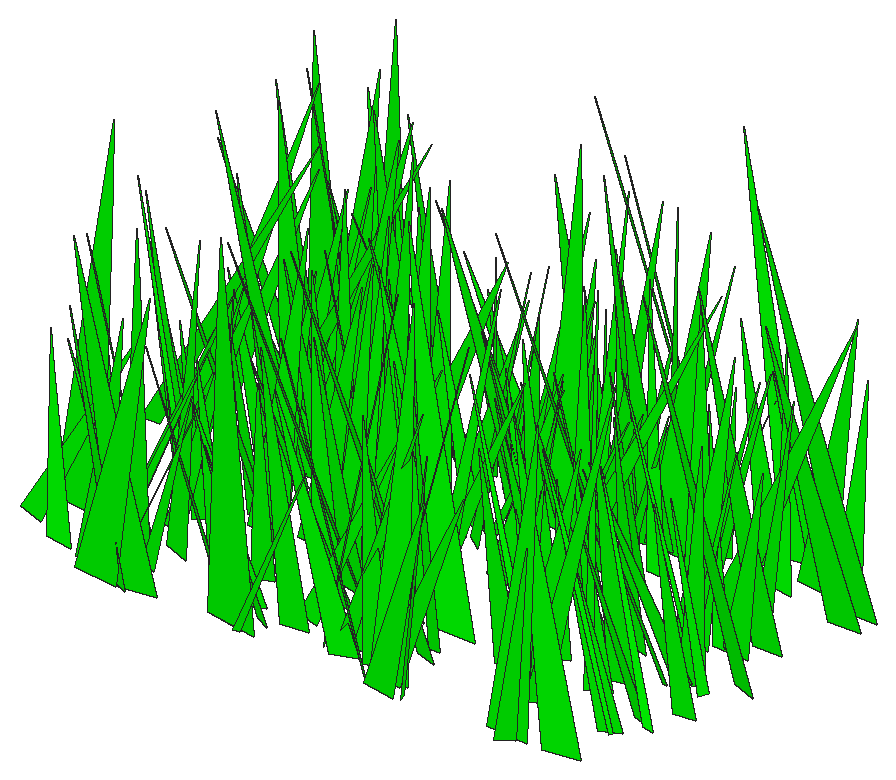
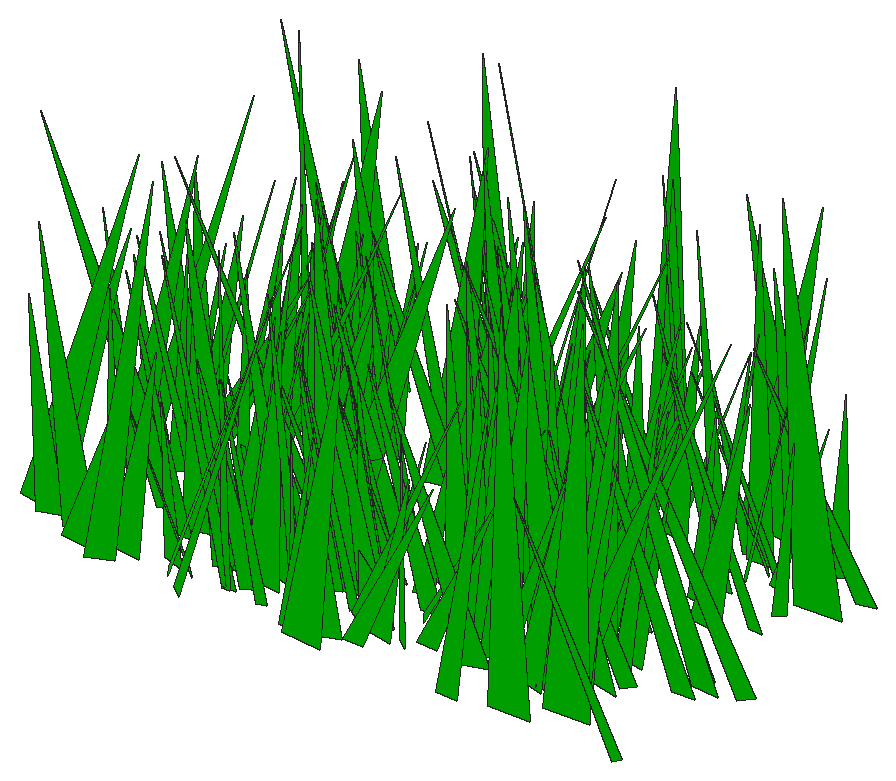
# SketchUp Ruby script. Lengths in inches.
U = 1.inch
M = Sketchup.active_model
def pt(a) = Geom::Point3d.new(a.map { |v| v * U })
def face(e, loops, mat)
  f = e.add_face(loops[0].map { |a| pt(a) })
  loops[1..].each { |l| e.add_face(l.map { |a| pt(a) }).erase! }
  f.material = f.back_material = mat if mat
  f
end
# faces: each face lists its corners as indices into pts; further lists are holes
def faces(e, pts, list, mat = nil) = list.each { |f| face(e, (f[0].is_a?(Array) ? f : [f]).map { |l| l.map { |i| pts[i] } }, mat) }
# xy, xz, yz: faces in a plane at the given z, y or x. An outline is a flat list of corners, or four numbers for a rectangle; further outlines are holes
def ring(l) = l.size == 4 ? [[l[0], l[1]], [l[2], l[1]], [l[2], l[3]], [l[0], l[3]]] : l.each_slice(2).to_a
def flat(e, list, mat, &to3) = list.each { |f| face(e, (f[0].is_a?(Array) ? f : [f]).map { |l| ring(l).map { |u, v| to3.(u, v) } }, mat) }
def xy(e, z, list, mat = nil) = flat(e, list, mat) { |x, y| [x, y, z] }
def xz(e, y, list, mat = nil) = flat(e, list, mat) { |x, z| [x, y, z] }
def yz(e, x, list, mat = nil) = flat(e, list, mat) { |y, z| [x, y, z] }
def lines(e, pts, list) = list.each { |a, b| e.add_line(pt(pts[a]), pt(pts[b])) }
# prism: a flat outline (further loops are holes) pulled along v
def prism(e, loops, v, mat = nil)
  f = face(e, loops, mat); d = Geom::Vector3d.new(v.map { |x| x * U })
  f.pushpull(f.normal.samedirection?(d) ? d.length : -d.length)
end
def box(e, o, s, mat = nil) = prism(e, [[o, [o[0] + s[0], o[1], o[2]], [o[0] + s[0], o[1] + s[1], o[2]], [o[0], o[1] + s[1], o[2]]]], [0, 0, s[2]], mat)
def at(x, y, z, deg = 0) = Geom::Transformation.translation(pt([x, y, z])) * Geom::Transformation.rotation(ORIGIN, Z_AXIS, deg.degrees)
def axes(o, x, y, z) = Geom::Transformation.new([*x, 0, *y, 0, *z, 0, *pt(o).to_a, 1])
def part(name) = M.definitions.add(name)
# library, detail: a bought-in or finely detailed component or shape, given as its bounding box
def library(name, o, s) = part(name).tap { |d| box(d.entities, o, s) }
def detail(e, o, s) = box(e.add_group.entities, o, s)
def put(e, d, t, mat = nil) = e.add_instance(d, t).tap { |i| i.material = mat if mat }
def group(e, t, mat = nil) = e.add_group.tap { |g| g.transformation = t; g.material = mat if mat }.entities
root = M.entities
M.materials.add("[0065_Lime]").color = [0, 255, 0]
c1 = part("fur_instance\#9")
p = [[0.8125,0,1.79],[0.67,-0.02,1.48],[0,-0.11,0],[0,0.11,0]]
faces(c1.entities,p,[[0,1,2,3]])
put(root,c1,axes([28.72,22.77,1.48],[-3.5361,0.35357,0.62096],[-2.38381,-0.50693,0.69047],[1.10969,0.03769,3.46199]),"[0065_Lime]")
put(root,c1,axes([28.78,19.72,1.48],[-2.9775,0.57338,0.01359],[-3.98278,-0.409,0.88436],[0.88789,0.0882,4.01253]),"[0065_Lime]")
put(root,c1,axes([27.87,21.88,1.48],[1.59134,1.15221,2.92207],[-8.95191,0.2009,0.57103],[0.06821,-0.51425,6.7702]),"[0065_Lime]")
put(root,c1,axes([29.9,21.47,1.48],[-3.74921,0.205,0.84488],[-1.69704,-0.51484,-0.79677],[0.572,-0.18381,3.17391]),"[0065_Lime]")
put(root,c1,axes([26.9,33.24,1.48],[5.29508,-0.1762,0.18665],[1.27098,0.7403,-0.43903],[-0.09771,0.08126,4.40438]),"[0065_Lime]")
put(root,c1,axes([26.95,20.6,1.48],[3.52402,0.60278,0.02909],[-4.2165,0.4855,0.855],[0.78993,-0.09757,4.43406]),"[0065_Lime]")
put(root,c1,axes([30.1,24.78,1.48],[-1.53905,0.72746,1.23673],[-5.38247,-0.19147,-0.65785],[-0.37698,-0.23612,4.34366]),"[0065_Lime]")
put(root,c1,axes([30.03,24.65,1.48],[-4.90512,-0.53874,1.71755],[4.17986,-0.70878,0.44836],[1.29866,0.24644,5.04419]),"[0065_Lime]")
put(root,c1,axes([30.4375,24.15,1.48],[-6.75899,0.10318,1.4523],[-0.56299,-0.97914,0.59733],[1.84661,0.07913,5.49784]),"[0065_Lime]")
put(root,c1,axes([27.95,27.57,1.48],[1.90571,-0.57874,0.3586],[4.07605,0.24988,-0.81846],[0.73696,0.11448,3.5995]),"[0065_Lime]")
put(root,c1,axes([30.14,31.13,1.48],[-4.8108,0.36742,1.63412],[-3.00649,-0.69382,-0.62879],[1.35421,-0.23512,4.40921]),"[0065_Lime]")
put(root,c1,axes([31.47,29.57,1.48],[-4.36689,-0.72132,0.39514],[5.15363,-0.60775,0.50828],[-0.16377,0.10881,5.45836]),"[0065_Lime]")
put(root,c1,axes([26.15,27.65,1.48],[8.05448,-0.36593,0.10917],[2.60265,1.12434,-0.76218],[0.16139,0.13106,6.84324]),"[0065_Lime]")
put(root,c1,axes([30.34,28.14,1.48],[-2.77665,0.35489,1.36449],[-2.98789,-0.37458,-0.75831],[0.51496,-0.25978,2.95745]),"[0065_Lime]")
put(root,c1,axes([30.97,21.69,1.48],[-6.33616,-0.14954,1.16675],[0.98148,-0.9122,-0.39106],[1.49221,-0.03497,5.21145]),"[0065_Lime]")
put(root,c1,axes([30.48,28.47,1.48],[-4.82918,-0.53417,1.11755],[3.75382,-0.70422,-0.54689],[1.4992,0.04263,4.96915]),"[0065_Lime]")
put(root,c1,axes([30.53,30.6,1.48],[-5.41771,-0.76266,1.43966],[5.44632,-0.79326,-0.52083],[1.7111,0.11017,6.21606]),"[0065_Lime]")
put(root,c1,axes([27.85,28.6875,1.48],[5.15808,0.64552,0.65599],[-4.66345,0.71658,0.63311],[-0.07723,-0.15712,5.58261]),"[0065_Lime]")
put(root,c1,axes([29.92,32,1.48],[-1.86684,-1.23711,0.9246],[8.83963,-0.27404,-0.47748],[0.81409,0.13867,7.30489]),"[0065_Lime]")
put(root,c1,axes([27.49,28.05,1.48],[7.17751,0.78944,0.96843],[-5.7172,1.00753,0.51447],[-0.54212,-0.17345,7.39622]),"[0065_Lime]")
put(root,c1,axes([28.67,24.05,1.48],[5.56756,-0.25053,0.07454],[1.75703,0.77643,0.61209],[-0.31607,-0.09682,4.7157]),"[0065_Lime]")
put(root,c1,axes([32.28,27.27,1.48],[-5.81157,-0.70001,1.7086],[5.33705,-0.81199,0.86353],[0.86294,0.30768,6.16607]),"[0065_Lime]")
put(root,c1,axes([30.13,29.91,1.48],[3.34774,0.73264,0.07321],[-5.18012,0.46896,-0.5325],[-0.59929,0.03912,5.0118]),"[0065_Lime]")
put(root,c1,axes([31.3125,23.7,1.48],[-3.40261,0.29121,1.77597],[-2.75556,-0.48772,-0.81322],[1.212,-0.2913,3.137]),"[0065_Lime]")
put(root,c1,axes([31.93,18.76,1.48],[-5.23082,-0.46131,0.97469],[3.16859,-0.75388,-0.70499],[1.47422,-0.01646,4.97365]),"[0065_Lime]")
put(root,c1,axes([32.09,31.2,1.48],[-2.31985,-0.60177,1.93],[4.89532,-0.29083,0.85459],[0.07595,0.36448,3.86846]),"[0065_Lime]")
put(root,c1,axes([30.48,19.34,1.48],[1.0224,-0.87725,0.57335],[6.26705,0.13534,-0.45547],[0.44254,0.11016,5.12558]),"[0065_Lime]")
put(root,c1,axes([32.7,30.59,1.48],[-7.74786,-0.11969,1.71735],[1.11795,-1.11673,0.72901],[1.98325,0.1619,6.29814]),"[0065_Lime]")
put(root,c1,axes([31.26,20.54,1.48],[4.80827,0.64677,3.01034],[-5.54314,0.72565,0.63379],[-2.03855,-0.44763,5.37703]),"[0065_Lime]")
put(root,c1,axes([32.66,18.77,1.48],[-1.21146,-1.0565,1.5288],[7.71905,-0.14063,0.79057],[-0.6918,0.28098,6.14398]),"[0065_Lime]")
put(root,c1,axes([32.08,27.91,1.48],[0.92743,-1.10638,2.25257],[8.30169,0.16274,0.41694],[-0.8625,0.37673,6.43525]),"[0065_Lime]")
put(root,c1,axes([33.12,31.41,1.48],[-4.13307,-0.46976,1.03758],[3.56684,-0.56267,0.86424],[0.2846,0.22982,4.23675]),"[0065_Lime]")
put(root,c1,axes([31.43,33.01,1.48],[-3.49602,-1.09361,2.3833],[8.09772,-0.54934,-0.58752],[1.89292,0.33024,6.91506]),"[0065_Lime]")
put(root,c1,axes([30.59,30.26,1.48],[5.59751,-0.2494,1.37056],[2.08303,0.79577,-0.77659],[-1.28457,0.20365,4.71293]),"[0065_Lime]")
put(root,c1,axes([33.59,27.43,1.48],[-2.81131,0.48483,0.02706],[-3.36983,-0.38449,-0.79968],[-0.74168,-0.0908,3.53078]),"[0065_Lime]")
put(root,c1,axes([30.1,21.04,1.48],[4.99048,0.28877,0.35872],[-2.08973,0.6988,0.3855],[-0.22515,-0.08529,4.37307]),"[0065_Lime]")
put(root,c1,axes([34.15,23.88,1.48],[-6.14823,-0.31663,0.55577],[2.32834,-0.85754,0.67122],[0.35091,0.14224,5.28389]),"[0065_Lime]")
put(root,c1,axes([30.93,31.15,1.48],[5.00355,-1.08655,0.74643],[7.72341,0.71202,0.47601],[-0.99127,0.06314,7.47653]),"[0065_Lime]")
put(root,c1,axes([30.68,20.86,1.48],[4.29098,0.08918,0.19069],[-0.58149,0.59423,-0.65508],[-0.34589,0.10737,3.46697]),"[0065_Lime]")
put(root,c1,axes([32.72,24.77,1.48],[-2.80205,-0.50191,0.49495],[3.53201,-0.40248,-0.44632],[0.80839,0.01877,3.66567]),"[0065_Lime]")
put(root,c1,axes([31.55,26.2,1.48],[0.82876,0.56028,0.01444],[-3.94864,0.11497,0.46315],[0.55391,-0.0187,3.28007]),"[0065_Lime]")
put(root,c1,axes([31.07,18.71,1.48],[1.54058,-1.05232,0.3585],[7.45525,0.20773,-0.7651],[0.83471,0.08688,6.17187]),"[0065_Lime]")
put(root,c1,axes([31.14,22.58,1.48],[4.95946,0.50295,1.09358],[-3.75844,0.6981,0.51904],[-0.70189,-0.1844,4.9478]),"[0065_Lime]")
put(root,c1,axes([32.09,21.51,1.48],[5.68742,0.51625,2.39145],[-4.26718,0.83899,0.64564],[-1.98301,-0.32476,5.46951]),"[0065_Lime]")
put(root,c1,axes([31.9375,20.31,1.48],[3.62474,0.29569,1.03947],[-2.38327,0.50159,0.71752],[-0.61742,-0.20021,3.33288]),"[0065_Lime]")
put(root,c1,axes([29.53,29.36,1.48],[8.42142,-0.30369,0.21284],[2.17439,1.18058,-0.47674],[-0.10711,0.08893,7.05599]),"[0065_Lime]")
put(root,c1,axes([33.83,30.46,1.48],[-4.81529,0.95459,0.64171],[-6.73172,-0.68549,0.74786],[1.20687,-0.01484,6.73179]),"[0065_Lime]")
put(root,c1,axes([33.67,33.36,1.48],[-5.15186,-0.62922,1.2017],[4.44942,-0.7505,-0.54693],[1.56092,0.06256,5.52527]),"[0065_Lime]")
put(root,c1,axes([34.57,20.59,1.48],[-4.89615,-0.12504,0.52726],[0.96937,-0.68647,0.50055],[0.5219,0.10196,4.01677]),"[0065_Lime]")
put(root,c1,axes([31.49,29.89,1.48],[5.60129,-0.86407,1.25797],[6.32205,0.78329,-0.59656],[-0.4859,0.23062,6.73952]),"[0065_Lime]")
put(root,c1,axes([32.66,25.73,1.48],[-1.28123,0.7327,1.5636],[-5.36847,-0.23483,0.77688],[1.43652,-0.22411,4.29789]),"[0065_Lime]")
put(root,c1,axes([33.58,28.07,1.48],[-3.70234,-0.61665,2.81856],[5.36388,-0.55661,0.58114],[1.57923,0.44487,4.63397]),"[0065_Lime]")
put(root,c1,axes([34.47,20.88,1.48],[1.58425,-0.6212,1.32415],[4.55005,0.26431,0.55305],[-1.22082,0.17896,3.7796]),"[0065_Lime]")
put(root,c1,axes([33.56,24.29,1.48],[0.88439,0.99039,1.1984],[-7.19374,0.11248,0.39757],[0.31229,-0.21366,5.76435]),"[0065_Lime]")
put(root,c1,axes([35.39,25.48,1.48],[-2.98273,-0.68462,1.34787],[5.14146,-0.40797,0.58425],[0.22049,0.25188,4.60985]),"[0065_Lime]")
put(root,c1,axes([33.07,28.9,1.48],[5.33723,-0.97526,0.63904],[6.9226,0.75708,0.46229],[-0.93024,0.03845,7.10671]),"[0065_Lime]")
put(root,c1,axes([34.9375,29.76,1.48],[-4.28948,0.66055,0.95634],[-4.63171,-0.62376,0.69147],[1.42395,-0.03907,5.12999]),"[0065_Lime]")
put(root,c1,axes([36.16,31.25,1.48],[-2.88799,0.47312,0.00249],[-3.34241,-0.40279,-0.4371],[-0.4059,-0.04948,3.58162]),"[0065_Lime]")
put(root,c1,axes([37.38,29.875,1.48],[-5.94972,-0.10522,0.01679],[0.74009,-0.82214,0.88385],[-0.11554,0.15185,4.79701]),"[0065_Lime]")
put(root,c1,axes([36.27,20.35,1.48],[-2.32592,0.50491,0.2701],[-3.57596,-0.31507,-0.6386],[-0.48366,-0.09863,3.42259]),"[0065_Lime]")
put(root,c1,axes([36.1,26.7,1.48],[-5.8963,-0.11837,1.20908],[0.5988,-0.84605,-0.84341],[1.60016,-0.11957,4.77085]),"[0065_Lime]")
put(root,c1,axes([35.86,28.8125,1.48],[0.5666,-1.20776,1.69318],[8.79229,0.10843,0.6451],[-0.95048,0.28308,6.97674]),"[0065_Lime]")
put(root,c1,axes([35.75,29.3,1.48],[1.10258,0.92393,0.21284],[-6.52192,0.15839,-0.68613],[-0.87547,-0.01635,5.37946]),"[0065_Lime]")
put(root,c1,axes([35.31,21.86,1.48],[2.47408,-0.61407,0.28859],[4.26838,0.35042,0.77422],[-1.00197,-0.02346,4.01073]),"[0065_Lime]")
put(root,c1,axes([35.86,28.45,1.48],[-4.21318,0.26406,1.69127],[-2.32385,-0.62403,-0.56551],[1.56659,-0.21552,3.70963]),"[0065_Lime]")
put(root,c1,axes([35.46,19.21,1.48],[6.90338,0.01171,2.27071],[0.22301,1.04031,-0.62834],[-2.78391,0.11237,5.58045]),"[0065_Lime]")
put(root,c1,axes([38.28,23.01,1.48],[-7.29496,-0.31664,0.22657],[2.2031,-1.01897,-0.78601],[0.54938,-0.11836,6.16053]),"[0065_Lime]")
put(root,c1,axes([34.12,31.34,1.48],[3.2239,-0.67529,0.07675],[4.76102,0.44643,-0.69802],[0.66075,0.07807,4.65512]),"[0065_Lime]")
put(root,c1,axes([37.03,19.67,1.48],[-3.52449,-0.30166,0.04655],[2.08957,-0.48527,-0.70038],[0.49576,-0.09925,3.28295]),"[0065_Lime]")
put(root,c1,axes([36.37,23.83,1.48],[-3.33471,0.69059,2.37133],[-5.58773,-0.49334,-0.38478],[1.19562,-0.37948,4.81564]),"[0065_Lime]")
put(root,c1,axes([36.03,19.03,1.48],[-2.69771,-0.90102,1.5194],[6.53677,-0.41426,-0.55272],[1.36942,0.20244,5.63147]),"[0065_Lime]")
put(root,c1,axes([35.21,24.59,1.48],[0.24312,-0.82666,1.95285],[6.27852,-0.02063,-0.80985],[0.97658,0.33845,4.72042]),"[0065_Lime]")
put(root,c1,axes([38.11,32.52,1.48],[-3.39189,0.46363,0.00651],[-3.27769,-0.47329,-0.44778],[-0.37814,-0.05623,3.82288]),"[0065_Lime]")
put(root,c1,axes([36.3,18.99,1.48],[-3.07127,-1.23304,1.14461],[8.75798,-0.45547,-0.89295],[1.50956,0.13379,7.50937]),"[0065_Lime]")
put(root,c1,axes([36.33,29.25,1.48],[-4.4804,0.75461,1.72832],[-5.34027,-0.6852,0.86516],[2.19892,-0.12652,5.62266]),"[0065_Lime]")
put(root,c1,axes([38.12,27.9,1.48],[-3.33452,-0.74369,0.8425],[5.38721,-0.45149,0.75292],[-0.24776,0.19206,5.03218]),"[0065_Lime]")
put(root,c1,axes([36.35,28,1.48],[5.99666,0.08389,1.90852],[-0.21962,0.89588,-0.86292],[-2.41108,0.12703,4.82532]),"[0065_Lime]")
put(root,c1,axes([38.42,22.09,1.48],[-3.87251,-0.50419,0.22774],[3.5912,-0.53754,0.52601],[-0.2363,0.09329,4.26187]),"[0065_Lime]")
put(root,c1,axes([36.45,27.32,1.48],[4.57674,0.51359,2.35356],[-4.2925,0.68652,0.50284],[-1.81804,-0.32801,4.73762]),"[0065_Lime]")
put(root,c1,axes([36.83,31.64,1.48],[4.25887,0.2267,1.4966],[-1.40147,0.65138,-0.66749],[-2.00595,0.02621,3.64381]),"[0065_Lime]")
put(root,c1,axes([36.5,27.79,1.48],[-3.589,0.86041,2.2665],[-6.42175,-0.5704,0.52778],[2.00448,-0.28685,5.74898]),"[0065_Lime]")
put(root,c1,axes([39.02,31.23,1.48],[-5.80078,-0.31348,0.56422],[2.32259,-0.80199,0.86783],[0.25245,0.17526,4.9803]),"[0065_Lime]")
put(root,c1,axes([37.71,31.74,1.48],[0.30036,0.57934,0.57781],[-4.07128,0.06351,-0.73363],[-0.96309,-0.08781,3.2815]),"[0065_Lime]")
put(root,c1,axes([38.02,20.04,1.48],[1.81678,0.74005,1.96243],[-5.56498,0.32164,-0.65572],[-1.60892,-0.27685,4.48395]),"[0065_Lime]")
put(root,c1,axes([38.35,28.68,1.48],[-3.14554,0.50459,0.05274],[-3.56846,-0.44046,0.39336],[0.4063,0.03796,3.8631]),"[0065_Lime]")
put(root,c1,axes([36.89,24.62,1.48],[-6.25067,0.53072,2.74807],[-3.7036,-0.99297,0.85218],[3.45864,-0.10414,5.87903]),"[0065_Lime]")
put(root,c1,axes([38.07,23.05,1.48],[-3.58353,-0.68054,0.41693],[4.77266,-0.50853,-0.67321],[0.9697,-0.01207,4.85414]),"[0065_Lime]")
put(root,c1,axes([36.9,23.99,1.48],[5.49947,-0.68316,1.31727],[4.8466,0.80183,0.54675],[-1.66411,0.07762,5.94563]),"[0065_Lime]")
put(root,c1,axes([37.44,25.22,1.48],[5.56364,1.01805,1.63954],[-7.2201,0.82166,-0.88547],[-2.10305,-0.12763,7.37739]),"[0065_Lime]")
put(root,c1,axes([38.96,29.94,1.48],[-3.5513,-0.26544,0.96159],[2.14498,-0.49191,0.69119],[0.60421,0.18613,3.19809]),"[0065_Lime]")
put(root,c1,axes([36.7,18.79,1.48],[4.27715,-0.09296,0.41345],[0.72331,0.59911,-0.43702],[-0.41574,0.08595,3.49323]),"[0065_Lime]")
put(root,c1,axes([40.58,23.0625,1.48],[-7.29683,-0.44608,0.32237],[3.12189,-1.02315,-0.6878],[0.6991,-0.087,6.43607]),"[0065_Lime]")
put(root,c1,axes([37.37,29.47,1.48],[2.83428,0.62215,0.79426],[-4.5335,0.38652,0.55846],[0.0662,-0.16747,4.23954]),"[0065_Lime]")
put(root,c1,axes([37.67,31.07,1.48],[5.36353,0.10664,1.19403],[-0.93308,0.77362,0.45793],[-1.36386,-0.1099,4.38236]),"[0065_Lime]")
put(root,c1,axes([36.97,24.11,1.48],[1.97069,0.7444,0.07462],[-5.20422,0.26938,0.89002],[0.99427,-0.06547,4.51063]),"[0065_Lime]")
put(root,c1,axes([40.37,19.63,1.48],[-1.89031,0.76108,0.06694],[-5.33542,-0.25948,-0.82906],[-0.93573,-0.05794,4.592]),"[0065_Lime]")
put(root,c1,axes([39.49,33.44,1.48],[0.22938,-0.98535,0.85706],[7.04804,0.04796,0.59973],[-0.77943,0.14373,5.67534]),"[0065_Lime]")
put(root,c1,axes([40.875,23.74,1.48],[-2.69535,0.98539,0.29612],[-7.01004,-0.37438,-0.47069],[-0.41055,-0.07681,6.09282]),"[0065_Lime]")
put(root,c1,axes([38.91,32.72,1.48],[-2.82008,0.53735,1.9113],[-4.06504,-0.4711,0.46973],[1.90276,-0.21004,3.83627]),"[0065_Lime]")
put(root,c1,axes([39.22,30.2,1.48],[-0.60579,-0.66776,0.84299],[4.80927,-0.10416,-0.47813],[0.72663,0.13268,3.86731]),"[0065_Lime]")
put(root,c1,axes([37.99,20.77,1.48],[3.76153,0.52015,0.16729],[-3.69528,0.52271,0.51501],[0.2989,-0.08358,4.26172]),"[0065_Lime]")
put(root,c1,axes([40.68,23.66,1.48],[-2.04476,0.66088,1.10482],[-4.89536,-0.27592,-0.46396],[-0.00293,-0.207,4.14565]),"[0065_Lime]")
put(root,c1,axes([41.6875,19.02,1.48],[-6.95907,-0.05614,1.00741],[0.56116,-0.98368,0.72806],[1.17412,0.13742,5.62298]),"[0065_Lime]")
put(root,c1,axes([40.47,33.04,1.48],[-4.02546,0.1987,1.20461],[-1.64443,-0.5872,-0.39031],[1.22004,-0.13587,3.44848]),"[0065_Lime]")
put(root,c1,axes([39.01,27.89,1.48],[6.34506,0.23684,1.53199],[-2.01871,0.90522,0.84266],[-1.52079,-0.21346,5.27324]),"[0065_Lime]")
put(root,c1,axes([40.08,33.06,1.48],[-3.58682,-0.28311,1.22965],[1.72526,-0.54544,-0.87832],[1.8352,-0.04055,3.229]),"[0065_Lime]")
put(root,c1,axes([39.38,30.05,1.48],[4.93183,0.80591,0.77487],[-5.71705,0.70416,-0.46525],[-1.05643,-0.04839,6.13515]),"[0065_Lime]")
put(root,c1,axes([39.42,30.84,1.48],[5.01325,-0.13726,1.02114],[1.1167,0.71909,-0.38842],[-1.13276,0.10141,4.13633]),"[0065_Lime]")
put(root,c1,axes([39.22,28.55,1.48],[3.98991,0.17878,0.30958],[-1.31259,0.55662,0.42183],[-0.20162,-0.08584,3.38023]),"[0065_Lime]")
put(root,c1,axes([42.14,22.83,1.48],[-4.68194,1.13728,0.03042],[-8.06271,-0.65591,0.64589],[0.706,0.05134,7.57804]),"[0065_Lime]")
put(root,c1,axes([40.32,32.46,1.48],[6.59305,-0.1941,2.1072],[1.75501,0.97795,-0.61461],[-2.35351,0.18551,5.44473]),"[0065_Lime]")
put(root,c1,axes([39.32,19.96,1.48],[8.53091,0.06369,1.77067],[-0.7424,1.22477,0.89031],[-2.09593,-0.17459,6.89167]),"[0065_Lime]")
put(root,c1,axes([40.68,30.18,1.48],[-3.98422,1.03163,2.37649],[-7.61061,-0.62465,0.64425],[2.12476,-0.30297,6.7639]),"[0065_Lime]")
put(root,c1,axes([43.13,26.73,1.48],[-4.6572,-0.95591,0.9855],[6.90582,-0.63696,0.88985],[-0.23403,0.22701,6.64664]),"[0065_Lime]")
put(root,c1,axes([40.21,28.1875,1.48],[-0.11964,-0.56067,1.10236],[4.09221,-0.06092,-0.74433],[1.00548,0.18121,3.16056]),"[0065_Lime]")
put(root,c1,axes([40.83,20.19,1.48],[-1.21884,0.633,0.29729],[-4.41637,-0.17811,0.72802],[0.96029,-0.01571,3.72552]),"[0065_Lime]")
put(root,c1,axes([40.71,30.3,1.48],[-3.04412,0.45262,1.80916],[-3.29809,-0.50982,0.60221],[2.10826,-0.144,3.55433]),"[0065_Lime]")
put(root,c1,axes([41.61,19.77,1.48],[2.65298,-0.698,1.21069],[4.99553,0.40703,0.62062],[-1.39085,0.13054,4.53842]),"[0065_Lime]")
put(root,c1,axes([42.49,21.12,1.48],[-3.56225,-0.47515,0.00564],[3.35004,-0.4961,-0.53747],[0.4599,-0.06668,3.95884]),"[0065_Lime]")
put(root,c1,axes([42.37,21.67,1.48],[-5.18262,-0.30047,1.88115],[2.62935,-0.75722,0.74012],[1.73411,0.25015,4.49986]),"[0065_Lime]")
put(root,c1,axes([40.62,24.05,1.48],[7.14365,-0.27839,1.8052],[2.2979,1.03154,-0.68592],[-1.88945,0.20199,5.99092]),"[0065_Lime]")
put(root,c1,axes([40.13,19.8125,1.48],[6.06577,-0.39062,0.42289],[2.7311,0.85398,0.51321],[-0.73417,-0.05054,5.40311]),"[0065_Lime]")
put(root,c1,axes([43.17,26.44,1.48],[-5.3278,-0.38862,0.60748],[2.6385,-0.752,-0.80951],[1.11571,-0.07739,4.81522]),"[0065_Lime]")
put(root,c1,axes([40.1,24.25,1.48],[5.07455,-0.45405,0.57749],[3.30639,0.7023,-0.72029],[-0.11341,0.15869,4.84018]),"[0065_Lime]")
put(root,c1,axes([42.72,31.375,1.48],[0.17583,0.88388,0.77574],[-6.32035,0.03959,-0.56383],[-0.7273,-0.13039,5.08735]),"[0065_Lime]")
put(root,c1,axes([42.78,26,1.48],[-4.27424,0.34598,0.9429],[-2.40403,-0.62216,0.43949],[1.27546,-0.01324,3.98818]),"[0065_Lime]")
put(root,c1,axes([43.18,26.04,1.48],[1.83392,0.45758,1.83763],[-3.492,0.35199,-0.63117],[-1.87448,-0.20805,2.9737]),"[0065_Lime]")
put(root,c1,axes([41.19,26.51,1.48],[1.02451,0.74226,0.27912],[-5.24299,0.13552,0.65643],[0.72925,-0.06844,4.32728]),"[0065_Lime]")
put(root,c1,axes([43.3,31.23,1.48],[-6.74881,-0.45341,2.21831],[3.69998,-0.98293,0.7157],[2.03937,0.28288,6.0425]),"[0065_Lime]")
put(root,c1,axes([44.52,33.43,1.48],[-7.55128,-0.20552,1.1546],[1.63178,-1.06826,0.68941],[1.22118,0.15659,6.21837]),"[0065_Lime]")
put(root,c1,axes([42.78,26.64,1.48],[0.75807,-0.59283,0.36814],[4.2019,0.11387,0.41954],[-0.58993,0.04925,3.46134]),"[0065_Lime]")
put(root,c1,axes([41.11,20.91,1.48],[7.39166,0.14226,1.26061],[-0.79806,1.05373,-0.8884],[-1.67027,0.12607,6.00322]),"[0065_Lime]")
put(root,c1,axes([41.91,32.4,1.48],[-3.25243,-0.36452,1.91854],[2.50631,-0.55785,-0.74039],[2.45171,0.08671,3.30201]),"[0065_Lime]")
put(root,c1,axes([45.56,32.55,1.48],[-9.33019,-0.10248,1.00207],[0.83611,-1.31657,0.63905],[1.1621,0.12445,7.58558]),"[0065_Lime]")
put(root,c1,axes([42.41,19.34,1.48],[-5.14413,0.86721,2.66672],[-6.40122,-0.81423,0.70276],[2.80368,-0.26787,6.49733]),"[0065_Lime]")
put(root,c1,axes([41.93,30.94,1.48],[5.97961,0.73342,1.14174],[-5.13432,0.86269,-0.77812],[-1.68858,-0.02592,6.4091]),"[0065_Lime]")
put(root,c1,axes([42.01,26.24,1.48],[4.56275,-0.3231,0.441],[2.17642,0.63935,0.79722],[-0.91871,-0.09003,4.07884]),"[0065_Lime]")
put(root,c1,axes([43.7,31.23,1.48],[-0.70874,-0.82472,1.11133],[6.01714,-0.08633,0.39228],[-0.32816,0.1983,4.7927]),"[0065_Lime]")
put(root,c1,axes([43.19,28.06,1.48],[4.8137,-0.56254,1.75254],[4.07986,0.72906,0.42729],[-2.00592,0.13289,5.07472]),"[0065_Lime]")
put(root,c1,axes([44.66,23.42,1.48],[-5.65329,0.14418,0.94489],[-0.94318,-0.80992,0.40743],[1.22987,0.04162,4.65579]),"[0065_Lime]")
put(root,c1,axes([42.18,28.1,1.48],[4.08923,-0.10754,0.42514],[0.87005,0.55991,-0.79126],[-0.31915,0.14855,3.29017]),"[0065_Lime]")
put(root,c1,axes([44.3,24.9375,1.48],[-0.39881,0.8813,0.93401],[-6.35277,-0.04111,-0.49485],[-0.54467,-0.16578,5.08788]),"[0065_Lime]")
put(root,c1,axes([43.41,32.32,1.48],[-6.45205,-0.33883,2.49665],[2.25258,-1.00371,-0.71285],[3.18764,0.02347,5.55717]),"[0065_Lime]")
put(root,c1,axes([42.61,18.56,1.48],[0.71259,-0.73988,0.25907],[5.19409,0.09054,-0.78856],[0.92042,0.06191,4.24943]),"[0065_Lime]")
put(root,c1,axes([46.46,26.48,1.48],[-8.01425,-0.28238,0.63707],[2.06375,-1.12705,0.43759],[0.62665,0.10036,6.70645]),"[0065_Lime]")
put(root,c1,axes([42.76,31.84,1.48],[2.90932,-0.50025,1.33003],[3.91523,0.38127,-0.86109],[-0.13687,0.27304,3.6393]),"[0065_Lime]")
put(root,c1,axes([45.33,26.05,1.48],[-2.7488,-0.64038,0.39409],[4.57553,-0.37895,0.48196],[-0.26078,0.10111,4.30215]),"[0065_Lime]")
put(root,c1,axes([43.48,18.69,1.48],[5.46637,-0.02086,1.50938],[-0.0173,0.80825,0.4158],[-1.86146,-0.06878,4.42858]),"[0065_Lime]")
put(root,c1,axes([42.88,28.99,1.48],[1.40457,-0.57808,0.27637],[4.07656,0.18632,-0.6487],[0.64911,0.08073,3.47596]),"[0065_Lime]")
put(root,c1,axes([42.48,19.17,1.48],[3.15607,-0.61969,0.14992],[4.3898,0.43736,-0.5667],[0.46051,0.07789,4.37461]),"[0065_Lime]")
put(root,c1,axes([43.33,30.26,1.48],[3.768,-0.23169,0.16489],[1.54529,0.51474,0.87255],[-0.60984,-0.12723,3.22976]),"[0065_Lime]")
put(root,c1,axes([44.83,22.35,1.48],[0.24966,-0.70648,0.57552],[5.04159,0.04627,0.45622],[-0.60056,0.09473,4.06913]),"[0065_Lime]")
put(root,c1,axes([44.77,29.88,1.48],[5.37827,-0.25437,2.67928],[2.58566,0.83683,-0.77193],[-2.7278,0.2917,4.55091]),"[0065_Lime]")
put(root,c1,axes([44.95,28.86,1.48],[-4.0824,-0.39773,0.73903],[2.64546,-0.585,-0.88091],[1.35599,-0.05614,3.94357]),"[0065_Lime]")
put(root,c1,axes([43.33,32.26,1.48],[6.72109,-0.26749,0.92063],[1.75193,0.95305,0.81661],[-1.35483,-0.09461,5.62309]),"[0065_Lime]")
put(root,c1,axes([44.02,31.22,1.48],[-2.63447,0.90986,2.46337],[-6.80648,-0.45785,0.85045],[2.1839,-0.3294,5.62217]),"[0065_Lime]")
put(root,c1,axes([42.49,28.2,1.48],[7.23785,0.53647,0.29768],[-3.83253,1.00751,0.8131],[0.14556,-0.14818,6.60633]),"[0065_Lime]")
put(root,c1,axes([45.74,32.0625,1.48],[2.17071,0.48918,0.18739],[-3.36351,0.30355,-0.77359],[-0.92685,0.0441,3.24619]),"[0065_Lime]")
put(root,c1,axes([45.92,23.7,1.48],[2.93996,-0.41056,0.89487],[2.82376,0.44026,0.63031],[-1.33171,0.02714,3.31206]),"[0065_Lime]")
put(root,c1,axes([45.53,22.14,1.48],[3.65789,-0.39969,0.64661],[2.75595,0.52586,0.57673],[-1.06174,-0.01204,3.72469]),"[0065_Lime]")
put(root,c1,axes([44.9,32.23,1.48],[4.10131,0.1116,0.20202],[-0.70423,0.55899,-0.88821],[-0.44332,0.1445,3.2799]),"[0065_Lime]")
put(root,c1,axes([46.41,30,1.48],[-3.30055,0.76912,0.78232],[-5.40307,-0.48089,0.75995],[1.30039,-0.04593,5.14319]),"[0065_Lime]")
put(root,c1,axes([47.73,33.3,1.48],[-7.82606,0.66379,1.73133],[-4.70549,-1.13735,0.53872],[2.16887,-0.07235,7.41607]),"[0065_Lime]")
put(root,c1,axes([47.4,32.49,1.48],[-0.71805,0.78047,0.02482],[-5.51395,-0.09964,-0.55132],[-0.66832,-0.01643,4.52199]),"[0065_Lime]")
put(root,c1,axes([45.78,22.33,1.48],[1.97562,-0.66537,1.84247],[5.24604,0.23882,-0.83192],[0.17709,0.34834,4.08967]),"[0065_Lime]")
put(root,c1,axes([48.03,23.94,1.48],[-6.36437,-0.07006,1.18895],[0.38961,-0.91565,-0.42807],[1.49442,-0.05965,5.17505]),"[0065_Lime]")
put(root,c1,axes([47.16,25.75,1.48],[-2.85766,-0.68924,0.39627],[4.79907,-0.4071,-0.82877],[1.12486,-0.01415,4.54254]),"[0065_Lime]")
put(root,c1,axes([48.18,22.875,1.48],[3.34907,-0.45855,1.96078],[3.44258,0.55361,0.44783],[-2.14675,0.17241,3.77709]),"[0065_Lime]")
put(root,c1,axes([48.29,20.7,1.48],[-3.48432,-0.23739,1.14641],[2.00602,-0.49512,0.59849],[0.90347,0.18383,3.09238]),"[0065_Lime]")
put(root,c1,axes([47.04,19.47,1.48],[-0.88841,0.76926,1.26403],[-5.57552,-0.16192,0.70917],[1.13956,-0.19248,4.45519]),"[0065_Lime]")
put(root,c1,axes([49.42,24.5,1.48],[-4.30724,-0.16453,0.21071],[1.19501,-0.60021,0.45799],[0.10003,0.08595,3.60171]),"[0065_Lime]")
put(root,c1,axes([46.5,30.51,1.48],[5.21018,-0.27598,0.6343],[1.90858,0.73972,0.41218],[-0.90714,-0.02879,4.51035]),"[0065_Lime]")
put(root,c1,axes([47.75,22.73,1.48],[8.26588,-0.05746,2.98969],[0.75643,1.26418,-0.56963],[-3.61998,0.13297,6.70766]),"[0065_Lime]")
put(root,c1,axes([48.32,23.77,1.48],[1.36027,-0.73856,0.91999],[5.2638,0.21631,0.66947],[-1.094,0.12248,4.3651]),"[0065_Lime]")
put(root,c1,axes([49.08,32.9,1.48],[-1.4424,0.57312,0.53145],[-4.08801,-0.18413,-0.68718],[-0.59185,-0.12492,3.45122]),"[0065_Lime]")
put(root,c1,axes([49.79,24.9375,1.48],[-2.70874,-0.54452,0.15421],[3.80229,-0.36612,0.86986],[-0.77139,0.10743,3.74613]),"[0065_Lime]")
put(root,c1,axes([47.54,18.89,1.48],[0.65254,-0.88603,2.82837],[7.19345,0.05822,-0.48691],[0.32278,0.49371,5.13332]),"[0065_Lime]")
put(root,c1,axes([47.71,18.56,1.48],[3.70721,-0.51474,0.2581],[3.55276,0.51778,0.8386],[-0.94722,-0.07252,4.15552]),"[0065_Lime]")
put(root,c1,axes([47.33,28.72,1.48],[5.57149,-0.14476,1.1729],[1.30237,0.7878,-0.83511],[-1.20182,0.18261,4.53245]),"[0065_Lime]")
put(root,c1,axes([49.6875,18.94,1.48],[-1.88596,0.98571,0.53679],[-7.03161,-0.25723,-0.51798],[-0.44681,-0.11253,5.88582]),"[0065_Lime]")
put(root,c1,axes([48.58,31.48,1.48],[4.50168,-0.26907,2.28362],[2.6918,0.682,-0.81818],[-2.07429,0.30108,3.8942]),"[0065_Lime]")
put(root,c1,axes([50.1,25.27,1.48],[-6.49008,0.00488,1.08106],[-0.15991,-0.9267,-0.49489],[1.31985,-0.08826,5.25594]),"[0065_Lime]")
put(root,c1,axes([50.12,21.09,1.48],[-5.71475,0.18446,0.99314],[-1.47254,-0.80991,-0.56554],[1.02258,-0.1354,4.73587]),"[0065_Lime]")
put(root,c1,axes([46.98,21.06,1.48],[7.40281,-0.54463,0.97442],[3.82157,1.05375,0.52637],[-1.36131,-0.00354,6.77653]),"[0065_Lime]")
put(root,c1,axes([49.97,21.06,1.48],[1.51937,-0.55466,1.97422],[4.22618,0.31306,0.79534],[-1.90033,0.25276,3.34723]),"[0065_Lime]")
put(root,c1,axes([49.35,27.4,1.48],[4.26909,-0.2252,2.36793],[2.37008,0.67313,-0.68204],[-2.3293,0.27218,3.64591]),"[0065_Lime]")
put(root,c1,axes([50.33,22.16,1.48],[-3.55831,-0.39237,0.0506],[2.7675,-0.49722,-0.43245],[0.37684,-0.05342,3.65368]),"[0065_Lime]")
put(root,c1,axes([48.42,27.08,1.48],[3.43968,-0.73257,2.32153],[5.90974,0.47084,-0.81485],[-0.6321,0.41565,5.01466]),"[0065_Lime]")
put(root,c1,axes([50.59,28.21,1.48],[4.05144,0.71252,3.48694],[-5.74893,0.7295,-0.57555],[-3.32242,-0.39342,5.24796]),"[0065_Lime]")
put(root,c1,axes([51.51,31.69,1.48],[-5.53747,-0.96123,1.12418],[6.96569,-0.7765,0.45375],[0.42893,0.20057,7.14449]),"[0065_Lime]")
put(root,c1,axes([50.81,21.92,1.48],[-5.33208,0.20934,0.81352],[-1.32503,-0.75649,0.77696],[1.20999,0.09411,4.43576]),"[0065_Lime]")
put(root,c1,axes([51.62,25.74,1.48],[-7.51063,-0.56807,0.9825],[4.00306,-1.0689,-0.46231],[1.33329,0.00924,6.92261]),"[0065_Lime]")
put(root,c1,axes([48.94,26.37,1.48],[4.86568,-0.06034,1.14086],[0.74123,0.69037,-0.86801],[-1.26577,0.17231,3.87721]),"[0065_Lime]")
put(root,c1,axes([51.55,30.91,1.48],[-2.56693,-0.89905,0.23772],[6.39629,-0.35757,0.38358],[-0.32949,0.06272,5.59439]),"[0065_Lime]")
put(root,c1,axes([49.32,32.24,1.48],[0.98084,-0.86933,1.76763],[6.53249,0.10277,-0.7047],[0.56868,0.31887,5.04617]),"[0065_Lime]")
put(root,c1,axes([50.78,24.74,1.48],[-3.98537,0.14541,1.28764],[-1.4634,-0.56577,-0.85582],[1.19804,-0.20736,3.23807]),"[0065_Lime]")
put(root,c1,axes([50.11,24.96,1.48],[3.74982,-0.64725,0.73138],[4.52425,0.54154,0.71145],[-1.2475,0.01844,4.77861]),"[0065_Lime]")
put(root,c1,axes([51.19,23.26,1.48],[0.73135,0.5696,1.60126],[-4.3879,0.15384,-0.5077],[-1.02628,-0.25182,3.3118]),"[0065_Lime]")
put(root,c1,axes([49.92,27.4375,1.48],[0.46448,-0.62169,0.8227],[4.50814,0.04673,-0.50074],[0.52328,0.14925,3.58372]),"[0065_Lime]")
put(root,c1,axes([47.95,29.38,1.48],[6.7998,-0.6617,0.37403],[4.73141,0.95068,-0.55426],[0.01179,0.1155,6.705]),"[0065_Lime]")
put(root,c1,axes([50.08,28.5,1.48],[4.40489,0.45435,1.64547],[-3.61466,0.63587,0.51884],[-1.21711,-0.2441,4.4143]),"[0065_Lime]")
put(root,c1,axes([50.77,31.97,1.48],[-2.02833,0.71531,0.30451],[-4.97608,-0.28972,0.87425],[1.13665,0.00811,4.3707]),"[0065_Lime]")
